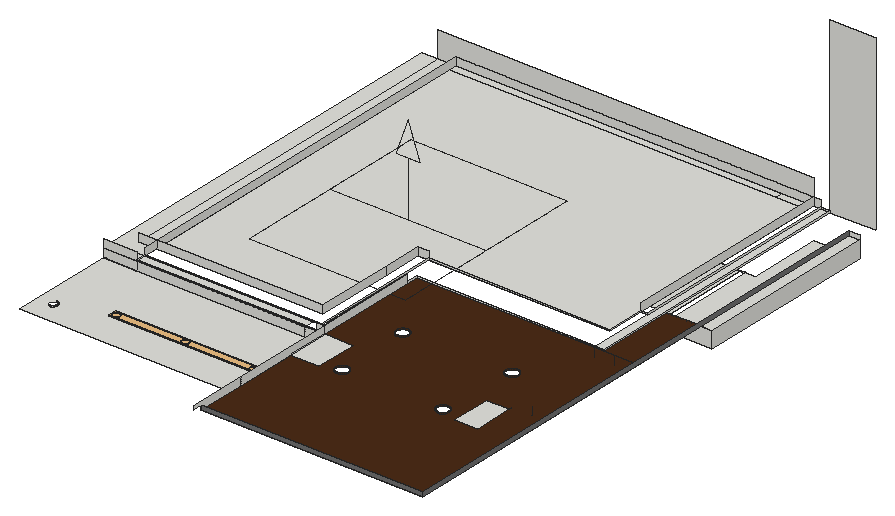
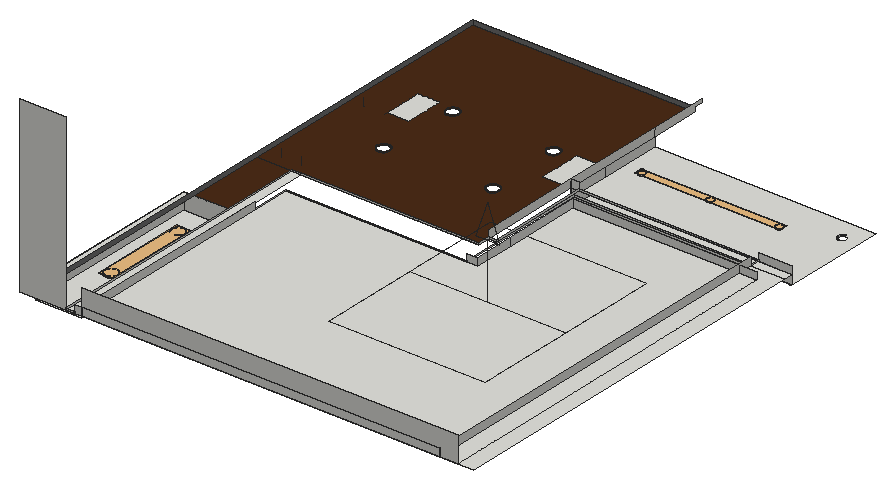
# SketchUp Ruby script. Lengths in inches.
U = 1.inch
M = Sketchup.active_model
def pt(a) = Geom::Point3d.new(a.map { |v| v * U })
def face(e, loops, mat)
  f = e.add_face(loops[0].map { |a| pt(a) })
  loops[1..].each { |l| e.add_face(l.map { |a| pt(a) }).erase! }
  f.material = f.back_material = mat if mat
  f
end
# faces: each face lists its corners as indices into pts; further lists are holes
def faces(e, pts, list, mat = nil) = list.each { |f| face(e, (f[0].is_a?(Array) ? f : [f]).map { |l| l.map { |i| pts[i] } }, mat) }
# xy, xz, yz: faces in a plane at the given z, y or x. An outline is a flat list of corners, or four numbers for a rectangle; further outlines are holes
def ring(l) = l.size == 4 ? [[l[0], l[1]], [l[2], l[1]], [l[2], l[3]], [l[0], l[3]]] : l.each_slice(2).to_a
def flat(e, list, mat, &to3) = list.each { |f| face(e, (f[0].is_a?(Array) ? f : [f]).map { |l| ring(l).map { |u, v| to3.(u, v) } }, mat) }
def xy(e, z, list, mat = nil) = flat(e, list, mat) { |x, y| [x, y, z] }
def xz(e, y, list, mat = nil) = flat(e, list, mat) { |x, z| [x, y, z] }
def yz(e, x, list, mat = nil) = flat(e, list, mat) { |y, z| [x, y, z] }
def lines(e, pts, list) = list.each { |a, b| e.add_line(pt(pts[a]), pt(pts[b])) }
# prism: a flat outline (further loops are holes) pulled along v
def prism(e, loops, v, mat = nil)
  f = face(e, loops, mat); d = Geom::Vector3d.new(v.map { |x| x * U })
  f.pushpull(f.normal.samedirection?(d) ? d.length : -d.length)
end
def box(e, o, s, mat = nil) = prism(e, [[o, [o[0] + s[0], o[1], o[2]], [o[0] + s[0], o[1] + s[1], o[2]], [o[0], o[1] + s[1], o[2]]]], [0, 0, s[2]], mat)
def at(x, y, z, deg = 0) = Geom::Transformation.translation(pt([x, y, z])) * Geom::Transformation.rotation(ORIGIN, Z_AXIS, deg.degrees)
def axes(o, x, y, z) = Geom::Transformation.new([*x, 0, *y, 0, *z, 0, *pt(o).to_a, 1])
def part(name) = M.definitions.add(name)
# library, detail: a bought-in or finely detailed component or shape, given as its bounding box
def library(name, o, s) = part(name).tap { |d| box(d.entities, o, s) }
def detail(e, o, s) = box(e.add_group.entities, o, s)
def put(e, d, t, mat = nil) = e.add_instance(d, t).tap { |i| i.material = mat if mat }
def group(e, t, mat = nil) = e.add_group.tap { |g| g.transformation = t; g.material = mat if mat }.entities
root = M.entities
M.materials.add("[Color M05]").color = [114, 114, 114]
M.materials.add("[Wood Veneer 01]").color = [76, 44, 23]
c1 = library("Group\#20",[-0.5,-0.5,-0.1],[139.5,7.875,0.2])
c2 = part("Group266\#1")
p = [[0,0,0],[0,0,-53.16],[-11.52,0,-53.16],[75.01,-97.09,0],[-75.01,-97.09,0],[75.01,97.09,0],
  [75.01,0,0],[-75.01,97.09,0],[11.52,0,-53.16],[-75.01,0,0],[0,0,-86.05]]
lines(c2.entities,p,[[0,1],[1,2],[3,4],[5,6],[7,5],[1,8],[9,0],[0,6],[8,10],[4,9],[6,3],[2,10],
  [9,7]])
c3 = part("Rectangle Light\#1")
put(c3.entities,c2,at(0,0,0))
c4 = library("Group\#22",[-0.5,-0.5,-0.1],[13.19,93.55,0.2])
xy(root,102.625,[[[3349.13,822.54,3349.13,844.85,3339.91,844.85,3339.91,929.47,3349.13,929.47,3349.13,999.35,3392.88,999.35,3392.88,822.54],[3374.07,926.86,3375.65,927.07,3377.12,927.68,3378.38,928.65,3379.35,929.91,3379.96,931.375,3380.16,932.95,3379.96,934.53,3379.35,936,3378.38,937.26,3377.12,938.23,3375.65,938.84,3374.07,939.05,3372.49,938.84,3371.02,938.23,3369.76,937.26,3368.79,936,3368.1875,934.53,3367.98,932.95,3368.1875,931.375,3368.79,929.91,3369.76,928.65,3371.02,927.68,3372.49,927.07],[3374.07,846.49,3375.625,846.7,3377.07,847.3,3378.3125,848.25,3379.27,849.49,3379.87,850.94,3380.07,852.49,3379.87,854.05,3379.27,855.49,3378.3125,856.74,3377.07,857.69,3375.625,858.29,3374.07,858.49,3372.52,858.29,3371.07,857.69,3369.83,856.74,3368.875,855.49,3368.28,854.05,3368.07,852.49,3368.28,850.94,3368.875,849.49,3369.83,848.25,3371.07,847.3,3372.52,846.7]],[3240.94,844.85,3334.66,928.79],[3334.66,844.85,3335.34,929.47],[3240.94,928.79,3334.66,929.47],[3335.34,928.79,3336.03,928.79,3336.03,928.91,3339.91,928.91,3339.91,929.47,3335.34,929.47],
  [3336.03,928.79,3339.91,928.91]])
xy(root,109.625,[[[2957.51,536.1875,3169.48,636.6875],[2972.07,553.83,2973.125,553.97,2974.1,554.38,2974.95,555.02,2975.59,555.87,2976,556.85,2976.14,557.9,2976,558.95,2975.59,559.93,2974.95,560.77,2974.1,561.42,2973.125,561.82,2972.07,561.96,2971.02,561.82,2970.04,561.42,2969.2,560.77,2968.55,559.93,2968.15,558.95,2968.01,557.9,2968.15,556.85,2968.55,555.87,2969.2,555.02,2970.04,554.38,2971.02,553.97],[3020.13,570.51,3021.02,570.63,3021.85,570.97,3022.56,571.52,3023.11,572.23,3023.45,573.0625,3023.57,573.95,3023.45,574.84,3023.11,575.67,3022.56,576.38,3021.85,576.93,3021.02,577.27,3020.13,577.39,3019.24,577.27,3018.41,576.93,3017.7,576.38,3017.15,575.67,3016.81,574.84,3016.69,573.95,3016.81,573.0625,3017.15,572.23,3017.7,571.52,3018.41,570.97,3019.24,570.63],[3085.94,570.51,3086.83,570.63,3087.66,570.97,3088.37,571.52,3088.92,572.23,3089.26,573.0625,3089.38,573.95,3089.26,574.84,3088.92,575.67,3088.37,576.38,3087.66,576.93,3086.83,577.27,3085.94,577.39,3085.05,577.27,3084.22,576.93,3083.51,576.38,3082.96,575.67,3082.62,574.84,3082.5,573.95,3082.62,573.0625,3082.96,572.23,3083.51,571.52,3084.22,570.97,3085.05,570.63],[3151.75,570.51,3152.64,570.63,3153.47,570.97,3154.19,571.52,3154.73,572.23,3155.07,573.0625,3155.19,573.95,3155.07,574.84,3154.73,575.67,3154.19,576.38,3153.47,576.93,3152.64,577.27,3151.75,577.39,3150.86,577.27,3150.04,576.93,3149.32,576.38,3148.78,575.67,3148.43,574.84,3148.32,573.95,3148.43,573.0625,3148.78,572.23,3149.32,571.52,3150.04,570.97,3150.86,570.63]]])
xy(root,118.5,[[3169.48,595.6875,3196.91,636.625],[3327.63,595.6875,3349.13,633.25],[2957.51,636.6875,2989.82,645.91],[2989.82,636.6875,3150.65,645.91],[2957.51,645.91,2989.82,645.91,2989.82,660.21,2972.24,660.21,2972.24,1019,2957.51,1019],
  [2972.24,660.21,2989.82,1019],[2989.82,660.21,2989.82,1011.63,3333.43,1011.63,3333.43,774.3125,3149.44,774.3125,3149.44,660.21],[3339.91,747.5625,3349.13,1019],[3382.57,822.54,3392.88,999.35],[2989.82,1011.63,3302.57,1019],
  [3302.57,1011.63,3333.43,1019]])
xy(root,118.5,[[[3169.48,488.8125,3169.48,595.6875,3196.91,595.6875,3196.91,636.625,3169.48,636.625,3169.48,747.5625,3382.57,747.5625,3382.57,488.8125],[3327.63,595.6875,3349.13,633.25],[3311.11,595.88,3312.66,596.09,3314.11,596.69,3315.35,597.64,3316.31,598.88,3316.91,600.33,3317.11,601.88,3316.91,603.43,3316.31,604.88,3315.35,606.125,3314.11,607.08,3312.66,607.68,3311.11,607.88,3309.56,607.68,3308.11,607.08,3306.87,606.125,3305.92,604.88,3305.32,603.43,3305.11,601.88,3305.32,600.33,3305.92,598.88,3306.87,597.64,3308.11,596.69,3309.56,596.09],[3214.3,668.63,3215.85,668.84,3217.3,669.44,3218.54,670.39,3219.5,671.63,3220.09,673.08,3220.3,674.63,3220.09,676.18,3219.5,677.63,3218.54,678.875,3217.3,679.83,3215.85,680.43,3214.3,680.63,3212.75,680.43,3211.3,679.83,3210.06,678.875,3209.1,677.63,3208.5,676.18,3208.3,674.63,3208.5,673.08,3209.1,671.63,3210.06,670.39,3211.3,669.44,3212.75,668.84],[3214.3,595.88,3215.85,596.09,3217.3,596.69,3218.54,597.64,3219.5,598.88,3220.09,600.33,3220.3,601.88,3220.09,603.43,3219.5,604.88,3218.54,606.125,3217.3,607.08,3215.85,607.68,3214.3,607.88,3212.75,607.68,3211.3,607.08,3210.06,606.125,3209.1,604.88,3208.5,603.43,3208.3,601.88,3208.5,600.33,3209.1,598.88,3210.06,597.64,3211.3,596.69,3212.75,596.09],[3316.66,671.87,3318.21,672.07,3319.66,672.67,3320.9,673.625,3321.86,674.87,3322.46,676.3125,3322.66,677.87,3322.46,679.42,3321.86,680.87,3320.9,682.11,3319.66,683.0625,3318.21,683.66,3316.66,683.87,3315.11,683.66,3313.66,683.0625,3312.42,682.11,3311.46,680.87,3310.87,679.42,3310.66,677.87,3310.87,676.3125,3311.46,674.87,3312.42,673.625,3313.66,672.67,3315.11,672.07]],[3349.13,747.5625,3382.57,822.54]],"[Wood Veneer 01]")
xz(root,488.8125,[[3169.48,118.5,3382.57,122.875]],"[Color M05]")
xz(root,636.6875,[[2957.51,109.5,2989.82,109.625],[2957.51,109.625,2989.82,118.5],[2989.82,109.625,3150.65,118.5],[3150.65,109.625,3169.48,118.5],[2957.51,118.5,2989.82,126],
  [2989.82,118.5,3162.07,119.75],[3162.07,118.5,3169.48,126]])
xz(root,645.91,[[2989.82,118.5,3159.13,119.75]])
xz(root,660.21,[[2972.24,118.5,3149.44,126]])
xz(root,735.75,[[3162.07,118.5,3169.48,119.75]])
xz(root,747.5625,[[3169.48,118.5,3339.91,119.75],[3339.91,118.5,3349.13,119.75]])
xz(root,774.3125,[[3149.44,118.5,3159.13,126],[3159.13,118.5,3333.43,119.75]])
xz(root,811.54,[[3333.43,118.5,3339.91,119.75]])
xz(root,822.54,[[3349.13,102.625,3392.88,118.5]])
xz(root,999.35,[[3382.57,118.5,3392.88,122.875]])
xz(root,1019,[[2972.24,118.5,2972.24,142.875,3333.43,142.875,3333.43,126,2989.82,126,2989.82,118.5],[2989.82,118.5,3333.43,126],[3333.43,118.5,3339.91,126],[3339.91,118.5,3349.13,119.75],[3349.13,118.5,3392.88,283.9375]])
yz(root,2989.82,[[636.6875,118.5,645.91,119.75],[645.91,118.5,1019,126]])
yz(root,3149.44,[[660.21,118.5,735.75,126],[735.75,118.5,774.3125,126]])
yz(root,3159.13,[[645.91,118.5,774.3125,119.75]])
yz(root,3162.07,[[636.6875,118.5,735.75,119.75]])
yz(root,3169.48,[[536.1875,109.625,595.6875,118.5],[595.6875,109.625,636.625,118.5],[636.625,109.625,636.6875,118.5],[488.8125,118.5,488.8125,122.875,479.5,122.875,479.5,126,536.1875,126,536.1875,118.5],[536.1875,118.5,636.6875,126],
  [636.6875,118.5,735.75,126],[735.75,118.5,747.5625,119.75]])
yz(root,3333.43,[[774.3125,118.5,811.54,119.75],[811.54,118.5,1019,126]])
yz(root,3339.91,[[811.54,118.5,1019,119.75]])
yz(root,3349.13,[[747.5625,118.5,1019,119.75]])
yz(root,3382.57,[[488.8125,118.5,999.35,122.875]],"[Color M05]")
yz(root,3392.88,[[822.54,102.625,999.35,118.5]])
p = [[3374.07,846.49,102.625],[3372.52,846.7,102.625],[3372.52,846.7,103.9375],[3374.07,846.49,103.9375],[3375.625,846.7,102.625],[3375.625,846.7,103.9375],
  [3371.07,847.3,102.625],[3371.07,847.3,103.9375],[3377.07,847.3,102.625],[3377.07,847.3,103.9375],[3369.83,848.25,102.625],[3369.83,848.25,103.9375],
  [3378.3125,848.25,102.625],[3378.3125,848.25,103.9375],[3368.875,849.49,102.625],[3368.875,849.49,103.9375],[3379.27,849.49,102.625],[3379.27,849.49,103.9375],
  [3368.28,850.94,102.625],[3368.28,850.94,103.9375],[3379.87,850.94,102.625],[3379.87,850.94,103.9375],[3368.07,852.49,102.625],[3368.07,852.49,103.9375],
  [3380.07,852.49,102.625],[3380.07,852.49,103.9375],[3368.28,854.05,102.625],[3368.28,854.05,103.9375],[3379.87,854.05,102.625],[3379.87,854.05,103.9375],
  [3368.875,855.49,102.625],[3368.875,855.49,103.9375],[3379.27,855.49,102.625],[3379.27,855.49,103.9375],[3369.83,856.74,102.625],[3369.83,856.74,103.9375],
  [3378.3125,856.74,102.625],[3378.3125,856.74,103.9375],[3371.07,857.69,102.625],[3371.07,857.69,103.9375],[3377.07,857.69,102.625],[3377.07,857.69,103.9375],
  [3372.52,858.29,102.625],[3372.52,858.29,103.9375],[3375.625,858.29,102.625],[3375.625,858.29,103.9375],[3374.07,858.49,102.625],[3374.07,858.49,103.9375],
  [3374.07,926.86,102.625],[3372.49,927.07,102.625],[3372.49,927.07,103.9375],[3374.07,926.86,103.9375],[3375.65,927.07,102.625],[3375.65,927.07,103.9375],
  [3371.02,927.68,102.625],[3371.02,927.68,103.9375],[3377.12,927.68,102.625],[3377.12,927.68,103.9375],[3369.76,928.65,102.625],[3369.76,928.65,103.9375],
  [3378.38,928.65,102.625],[3378.38,928.65,103.9375],[3368.79,929.91,102.625],[3368.79,929.91,103.9375],[3379.35,929.91,102.625],[3379.35,929.91,103.9375],
  [3368.1875,931.375,102.625],[3368.1875,931.375,103.9375],[3379.96,931.375,102.625],[3379.96,931.375,103.9375],[3367.98,932.95,102.625],[3367.98,932.95,103.9375],
  [3380.16,932.95,102.625],[3380.16,932.95,103.9375],[3368.1875,934.53,102.625],[3368.1875,934.53,103.9375],[3379.96,934.53,102.625],[3379.96,934.53,103.9375],
  [3368.79,936,102.625],[3368.79,936,103.9375],[3379.35,936,102.625],[3379.35,936,103.9375],[3369.76,937.26,102.625],[3369.76,937.26,103.9375],
  [3378.38,937.26,102.625],[3378.38,937.26,103.9375],[3371.02,938.23,102.625],[3371.02,938.23,103.9375],[3377.12,938.23,102.625],[3377.12,938.23,103.9375],
  [3372.49,938.84,102.625],[3372.49,938.84,103.9375],[3375.65,938.84,102.625],[3375.65,938.84,103.9375],[3374.07,939.05,102.625],[3374.07,939.05,103.9375],
  [2973.125,553.97,109.625],[2972.07,553.83,109.625],[2972.07,553.83,110.5625],[2973.125,553.97,110.5625],[2974.1,554.38,109.625],[2974.1,554.38,110.5625],
  [2974.95,555.02,109.625],[2974.95,555.02,110.5625],[2975.59,555.87,109.625],[2975.59,555.87,110.5625],[2976,556.85,109.625],[2976,556.85,110.5625],
  [2976.14,557.9,109.625],[2976.14,557.9,110.5625],[2976,558.95,109.625],[2976,558.95,110.5625],[2975.59,559.93,109.625],[2975.59,559.93,110.5625],
  [2974.95,560.77,109.625],[2974.95,560.77,110.5625],[2974.1,561.42,109.625],[2974.1,561.42,110.5625],[2973.125,561.82,109.625],[2973.125,561.82,110.5625],
  [2972.07,561.96,109.625],[2972.07,561.96,110.5625],[3020.13,570.51,109.625],[3019.24,570.63,109.625],[3019.24,570.63,110.0625],[3020.13,570.51,110.0625],
  [3021.02,570.63,109.625],[3021.02,570.63,110.0625],[3085.94,570.51,109.625],[3085.05,570.63,109.625],[3085.05,570.63,110.0625],[3085.94,570.51,110.0625],
  [3086.83,570.63,109.625],[3086.83,570.63,110.0625],[3151.75,570.51,109.625],[3150.86,570.63,109.625],[3150.86,570.63,110.0625],[3151.75,570.51,110.0625],
  [3152.64,570.63,109.625],[3152.64,570.63,110.0625],[3018.41,570.97,109.625],[3018.41,570.97,110.0625],[3021.85,570.97,109.625],[3021.85,570.97,110.0625],
  [3084.22,570.97,109.625],[3084.22,570.97,110.0625],[3087.66,570.97,109.625],[3087.66,570.97,110.0625],[3150.04,570.97,109.625],[3150.04,570.97,110.0625],
  [3153.47,570.97,109.625],[3153.47,570.97,110.0625],[3017.7,571.52,109.625],[3017.7,571.52,110.0625],[3022.56,571.52,109.625],[3022.56,571.52,110.0625],
  [3083.51,571.52,109.625],[3083.51,571.52,110.0625],[3088.37,571.52,109.625],[3088.37,571.52,110.0625],[3149.32,571.52,109.625],[3149.32,571.52,110.0625],
  [3154.19,571.52,109.625],[3154.19,571.52,110.0625],[3017.15,572.23,109.625],[3017.15,572.23,110.0625],[3023.11,572.23,109.625],[3023.11,572.23,110.0625],
  [3082.96,572.23,109.625],[3082.96,572.23,110.0625],[3088.92,572.23,109.625],[3088.92,572.23,110.0625],[3148.78,572.23,109.625],[3148.78,572.23,110.0625],
  [3154.73,572.23,109.625],[3154.73,572.23,110.0625],[3016.81,573.0625,109.625],[3016.81,573.0625,110.0625],[3023.45,573.0625,109.625],[3023.45,573.0625,110.0625],
  [3082.62,573.0625,109.625],[3082.62,573.0625,110.0625],[3089.26,573.0625,109.625],[3089.26,573.0625,110.0625],[3148.43,573.0625,109.625],[3148.43,573.0625,110.0625],
  [3155.07,573.0625,109.625],[3155.07,573.0625,110.0625],[3016.69,573.95,109.625],[3016.69,573.95,110.0625],[3023.57,573.95,109.625],[3023.57,573.95,110.0625],
  [3082.5,573.95,109.625],[3082.5,573.95,110.0625],[3089.38,573.95,109.625],[3089.38,573.95,110.0625],[3148.32,573.95,109.625],[3148.32,573.95,110.0625],
  [3155.19,573.95,109.625],[3155.19,573.95,110.0625],[3016.81,574.84,109.625],[3016.81,574.84,110.0625],[3023.45,574.84,109.625],[3023.45,574.84,110.0625],
  [3082.62,574.84,109.625],[3082.62,574.84,110.0625],[3089.26,574.84,109.625],[3089.26,574.84,110.0625],[3148.43,574.84,109.625],[3148.43,574.84,110.0625],
  [3155.07,574.84,109.625],[3155.07,574.84,110.0625],[3017.15,575.67,109.625],[3017.15,575.67,110.0625],[3023.11,575.67,109.625],[3023.11,575.67,110.0625],
  [3082.96,575.67,109.625],[3082.96,575.67,110.0625],[3088.92,575.67,109.625],[3088.92,575.67,110.0625],[3148.78,575.67,109.625],[3148.78,575.67,110.0625],
  [3154.73,575.67,109.625],[3154.73,575.67,110.0625],[3017.7,576.38,109.625],[3017.7,576.38,110.0625],[3022.56,576.38,109.625],[3022.56,576.38,110.0625],
  [3083.51,576.38,109.625],[3083.51,576.38,110.0625],[3088.37,576.38,109.625],[3088.37,576.38,110.0625],[3149.32,576.38,109.625],[3149.32,576.38,110.0625],
  [3154.19,576.38,109.625],[3154.19,576.38,110.0625],[3018.41,576.93,109.625],[3018.41,576.93,110.0625],[3021.85,576.93,109.625],[3021.85,576.93,110.0625],
  [3084.22,576.93,109.625],[3084.22,576.93,110.0625],[3087.66,576.93,109.625],[3087.66,576.93,110.0625],[3150.04,576.93,109.625],[3150.04,576.93,110.0625],
  [3153.47,576.93,109.625],[3153.47,576.93,110.0625],[3019.24,577.27,109.625],[3019.24,577.27,110.0625],[3021.02,577.27,109.625],[3021.02,577.27,110.0625],
  [3085.05,577.27,109.625],[3085.05,577.27,110.0625],[3086.83,577.27,109.625],[3086.83,577.27,110.0625],[3150.86,577.27,109.625],[3150.86,577.27,110.0625],
  [3152.64,577.27,109.625],[3152.64,577.27,110.0625],[3020.13,577.39,109.625],[3020.13,577.39,110.0625],[3085.94,577.39,109.625],[3085.94,577.39,110.0625],
  [3151.75,577.39,109.625],[3151.75,577.39,110.0625],[3214.3,595.88,118.5],[3212.75,596.09,118.5],[3212.75,596.09,119.375],[3214.3,595.88,119.375],
  [3215.85,596.09,118.5],[3215.85,596.09,119.375],[3311.11,595.88,118.5],[3309.56,596.09,118.5],[3309.56,596.09,119.375],[3311.11,595.88,119.375],
  [3312.66,596.09,118.5],[3312.66,596.09,119.375],[3211.3,596.69,118.5],[3211.3,596.69,119.375],[3217.3,596.69,118.5],[3217.3,596.69,119.375],
  [3308.11,596.69,118.5],[3308.11,596.69,119.375],[3314.11,596.69,118.5],[3314.11,596.69,119.375],[3210.06,597.64,118.5],[3210.06,597.64,119.375],
  [3218.54,597.64,118.5],[3218.54,597.64,119.375],[3306.87,597.64,118.5],[3306.87,597.64,119.375],[3315.35,597.64,118.5],[3315.35,597.64,119.375],
  [3209.1,598.88,118.5],[3209.1,598.88,119.375],[3219.5,598.88,118.5],[3219.5,598.88,119.375],[3305.92,598.88,118.5],[3305.92,598.88,119.375],
  [3316.31,598.88,118.5],[3316.31,598.88,119.375],[3208.5,600.33,118.5],[3208.5,600.33,119.375],[3220.09,600.33,118.5],[3220.09,600.33,119.375],
  [3305.32,600.33,118.5],[3305.32,600.33,119.375],[3316.91,600.33,118.5],[3316.91,600.33,119.375],[3208.3,601.88,118.5],[3208.3,601.88,119.375],
  [3220.3,601.88,118.5],[3220.3,601.88,119.375],[3305.11,601.88,118.5],[3305.11,601.88,119.375],[3317.11,601.88,118.5],[3317.11,601.88,119.375],
  [3208.5,603.43,118.5],[3208.5,603.43,119.375],[3220.09,603.43,118.5],[3220.09,603.43,119.375],[3305.32,603.43,118.5],[3305.32,603.43,119.375],
  [3316.91,603.43,118.5],[3316.91,603.43,119.375],[3209.1,604.88,118.5],[3209.1,604.88,119.375],[3219.5,604.88,118.5],[3219.5,604.88,119.375],
  [3305.92,604.88,118.5],[3305.92,604.88,119.375],[3316.31,604.88,118.5],[3316.31,604.88,119.375],[3210.06,606.125,118.5],[3210.06,606.125,119.375],
  [3218.54,606.125,118.5],[3218.54,606.125,119.375],[3306.87,606.125,118.5],[3306.87,606.125,119.375],[3315.35,606.125,118.5],[3315.35,606.125,119.375],
  [3211.3,607.08,118.5],[3211.3,607.08,119.375],[3217.3,607.08,118.5],[3217.3,607.08,119.375],[3308.11,607.08,118.5],[3308.11,607.08,119.375],
  [3314.11,607.08,118.5],[3314.11,607.08,119.375],[3212.75,607.68,118.5],[3212.75,607.68,119.375],[3215.85,607.68,118.5],[3215.85,607.68,119.375],
  [3309.56,607.68,118.5],[3309.56,607.68,119.375],[3312.66,607.68,118.5],[3312.66,607.68,119.375],[3214.3,607.88,118.5],[3214.3,607.88,119.375],
  [3311.11,607.88,118.5],[3311.11,607.88,119.375],[3214.3,668.63,118.5],[3212.75,668.84,118.5],[3212.75,668.84,119.375],[3214.3,668.63,119.375],
  [3215.85,668.84,118.5],[3215.85,668.84,119.375],[3211.3,669.44,118.5],[3211.3,669.44,119.375],[3217.3,669.44,118.5],[3217.3,669.44,119.375],
  [3210.06,670.39,118.5],[3210.06,670.39,119.375],[3218.54,670.39,118.5],[3218.54,670.39,119.375],[3209.1,671.63,118.5],[3209.1,671.63,119.375],
  [3219.5,671.63,118.5],[3219.5,671.63,119.375],[3208.5,673.08,118.5],[3208.5,673.08,119.375],[3220.09,673.08,118.5],[3220.09,673.08,119.375],
  [3316.66,671.87,118.5],[3315.11,672.07,118.5],[3315.11,672.07,119.375],[3316.66,671.87,119.375],[3318.21,672.07,118.5],[3318.21,672.07,119.375],
  [3313.66,672.67,118.5],[3313.66,672.67,119.375],[3319.66,672.67,118.5],[3319.66,672.67,119.375],[3312.42,673.625,118.5],[3312.42,673.625,119.375],
  [3320.9,673.625,118.5],[3320.9,673.625,119.375],[3208.3,674.63,118.5],[3208.3,674.63,119.375],[3220.3,674.63,118.5],[3220.3,674.63,119.375],
  [3311.46,674.87,118.5],[3311.46,674.87,119.375],[3321.86,674.87,118.5],[3321.86,674.87,119.375],[3208.5,676.18,118.5],[3208.5,676.18,119.375],
  [3220.09,676.18,118.5],[3220.09,676.18,119.375],[3310.87,676.3125,118.5],[3310.87,676.3125,119.375],[3322.46,676.3125,118.5],[3322.46,676.3125,119.375],
  [3209.1,677.63,118.5],[3209.1,677.63,119.375],[3219.5,677.63,118.5],[3219.5,677.63,119.375],[3310.66,677.87,118.5],[3310.66,677.87,119.375],
  [3322.66,677.87,118.5],[3322.66,677.87,119.375],[3210.06,678.875,118.5],[3210.06,678.875,119.375],[3218.54,678.875,118.5],[3218.54,678.875,119.375],
  [3310.87,679.42,118.5],[3310.87,679.42,119.375],[3322.46,679.42,118.5],[3322.46,679.42,119.375],[3211.3,679.83,118.5],[3211.3,679.83,119.375],
  [3217.3,679.83,118.5],[3217.3,679.83,119.375],[3311.46,680.87,118.5],[3311.46,680.87,119.375],[3321.86,680.87,118.5],[3321.86,680.87,119.375],
  [3212.75,680.43,118.5],[3212.75,680.43,119.375],[3215.85,680.43,118.5],[3215.85,680.43,119.375],[3214.3,680.63,118.5],[3214.3,680.63,119.375],
  [3312.42,682.11,118.5],[3312.42,682.11,119.375],[3320.9,682.11,118.5],[3320.9,682.11,119.375],[3313.66,683.0625,118.5],[3313.66,683.0625,119.375],
  [3319.66,683.0625,118.5],[3319.66,683.0625,119.375],[3315.11,683.66,118.5],[3315.11,683.66,119.375],[3318.21,683.66,118.5],[3318.21,683.66,119.375],
  [3316.66,683.87,118.5],[3316.66,683.87,119.375],[3349.13,636.625,118.5],[3349.13,633.25,118.5],[3368.57,636.6875,118.5],[3368.57,636.6875,126],
  [3368.57,636.625,118.5],[3368.57,735.75,126],[3368.57,735.75,118.5],[3349.13,735.75,126],[3349.13,735.75,118.5]]
faces(root,p,[[0,1,2,3],[4,0,3,5],[1,6,7,2],[8,4,5,9],[6,10,11,7],[12,8,9,13],[10,14,15,11],[16,12,13,17],
  [14,18,19,15],[20,16,17,21],[18,22,23,19],[24,20,21,25],[22,26,27,23],[28,24,25,29],[26,30,31,27],[32,28,29,33],
  [30,34,35,31],[36,32,33,37],[34,38,39,35],[40,36,37,41],[38,42,43,39],[44,40,41,45],[42,46,47,43],[46,44,45,47],
  [48,49,50,51],[52,48,51,53],[49,54,55,50],[56,52,53,57],[54,58,59,55],[60,56,57,61],[58,62,63,59],[64,60,61,65],
  [62,66,67,63],[68,64,65,69],[66,70,71,67],[72,68,69,73],[70,74,75,71],[76,72,73,77],[74,78,79,75],[80,76,77,81],
  [78,82,83,79],[84,80,81,85],[82,86,87,83],[88,84,85,89],[86,90,91,87],[92,88,89,93],[90,94,95,91],[94,92,93,95],
  [96,97,98,99],[100,96,99,101],[102,100,101,103],[104,102,103,105],[106,104,105,107],[108,106,107,109],[110,108,109,111],[112,110,111,113],
  [114,112,113,115],[116,114,115,117],[118,116,117,119],[120,118,119,121],[122,123,124,125],[126,122,125,127],[128,129,130,131],[132,128,131,133],
  [134,135,136,137],[138,134,137,139],[123,140,141,124],[142,126,127,143],[129,144,145,130],[146,132,133,147],[135,148,149,136],[150,138,139,151],
  [140,152,153,141],[154,142,143,155],[144,156,157,145],[158,146,147,159],[148,160,161,149],[162,150,151,163],[152,164,165,153],[166,154,155,167],
  [156,168,169,157],[170,158,159,171],[160,172,173,161],[174,162,163,175],[164,176,177,165],[178,166,167,179],[168,180,181,169],[182,170,171,183],
  [172,184,185,173],[186,174,175,187],[176,188,189,177],[190,178,179,191],[180,192,193,181],[194,182,183,195],[184,196,197,185],[198,186,187,199],
  [188,200,201,189],[202,190,191,203],[192,204,205,193],[206,194,195,207],[196,208,209,197],[210,198,199,211],[200,212,213,201],[214,202,203,215],
  [204,216,217,205],[218,206,207,219],[208,220,221,209],[222,210,211,223],[212,224,225,213],[226,214,215,227],[216,228,229,217],[230,218,219,231],
  [220,232,233,221],[234,222,223,235],[224,236,237,225],[238,226,227,239],[228,240,241,229],[242,230,231,243],[232,244,245,233],[246,234,235,247],
  [236,248,249,237],[250,238,239,251],[240,252,253,241],[254,242,243,255],[244,256,257,245],[258,246,247,259],[248,260,261,249],[260,250,251,261],
  [252,262,263,253],[262,254,255,263],[256,264,265,257],[264,258,259,265]])
faces(root,p,[[266,267,268,269],[270,266,269,271],[272,273,274,275],[276,272,275,277],[267,278,279,268],[280,270,271,281],[273,282,283,274],[284,276,277,285],
  [278,286,287,279],[288,280,281,289],[282,290,291,283],[292,284,285,293],[286,294,295,287],[296,288,289,297],[290,298,299,291],[300,292,293,301],
  [294,302,303,295],[304,296,297,305],[298,306,307,299],[308,300,301,309],[302,310,311,303],[312,304,305,313],[306,314,315,307],[316,308,309,317],
  [310,318,319,311],[320,312,313,321],[314,322,323,315],[324,316,317,325],[318,326,327,319],[328,320,321,329],[322,330,331,323],[332,324,325,333],
  [326,334,335,327],[336,328,329,337],[330,338,339,331],[340,332,333,341],[334,342,343,335],[344,336,337,345],[338,346,347,339],[348,340,341,349],
  [342,350,351,343],[352,344,345,353],[346,354,355,347],[356,348,349,357],[350,358,359,351],[358,352,353,359],[354,360,361,355],[360,356,357,361],
  [362,363,364,365],[366,362,365,367],[363,368,369,364],[370,366,367,371],[368,372,373,369],[374,370,371,375],[372,376,377,373],[378,374,375,379],
  [376,380,381,377],[382,378,379,383],[384,385,386,387],[388,384,387,389],[385,390,391,386],[392,388,389,393],[390,394,395,391],[396,392,393,397],
  [380,398,399,381],[400,382,383,401],[394,402,403,395],[404,396,397,405],[398,406,407,399],[408,400,401,409],[402,410,411,403],[412,404,405,413],
  [406,414,415,407],[416,408,409,417],[410,418,419,411],[420,412,413,421],[414,422,423,415],[424,416,417,425],[418,426,427,419],[428,420,421,429],
  [422,430,431,423],[432,424,425,433],[426,434,435,427],[436,428,429,437],[430,438,439,431],[440,432,433,441],[438,442,443,439],[442,440,441,443],
  [434,444,445,435],[446,436,437,447],[444,448,449,445],[450,446,447,451],[448,452,453,449],[454,450,451,455],[452,456,457,453],[456,454,455,457]],"[Wood Veneer 01]")
lines(root,p,[[458,459],[460,461],[460,462],[463,464],[465,466]])
put(root,c1,at(3016.69,570.51,110.0625))
put(root,c3,axes([3109.1,812.42,118.51],[1,0,0],[0,1,0],[0,0,-1]))
put(root,c4,at(3367.98,846.49,103.9375))
